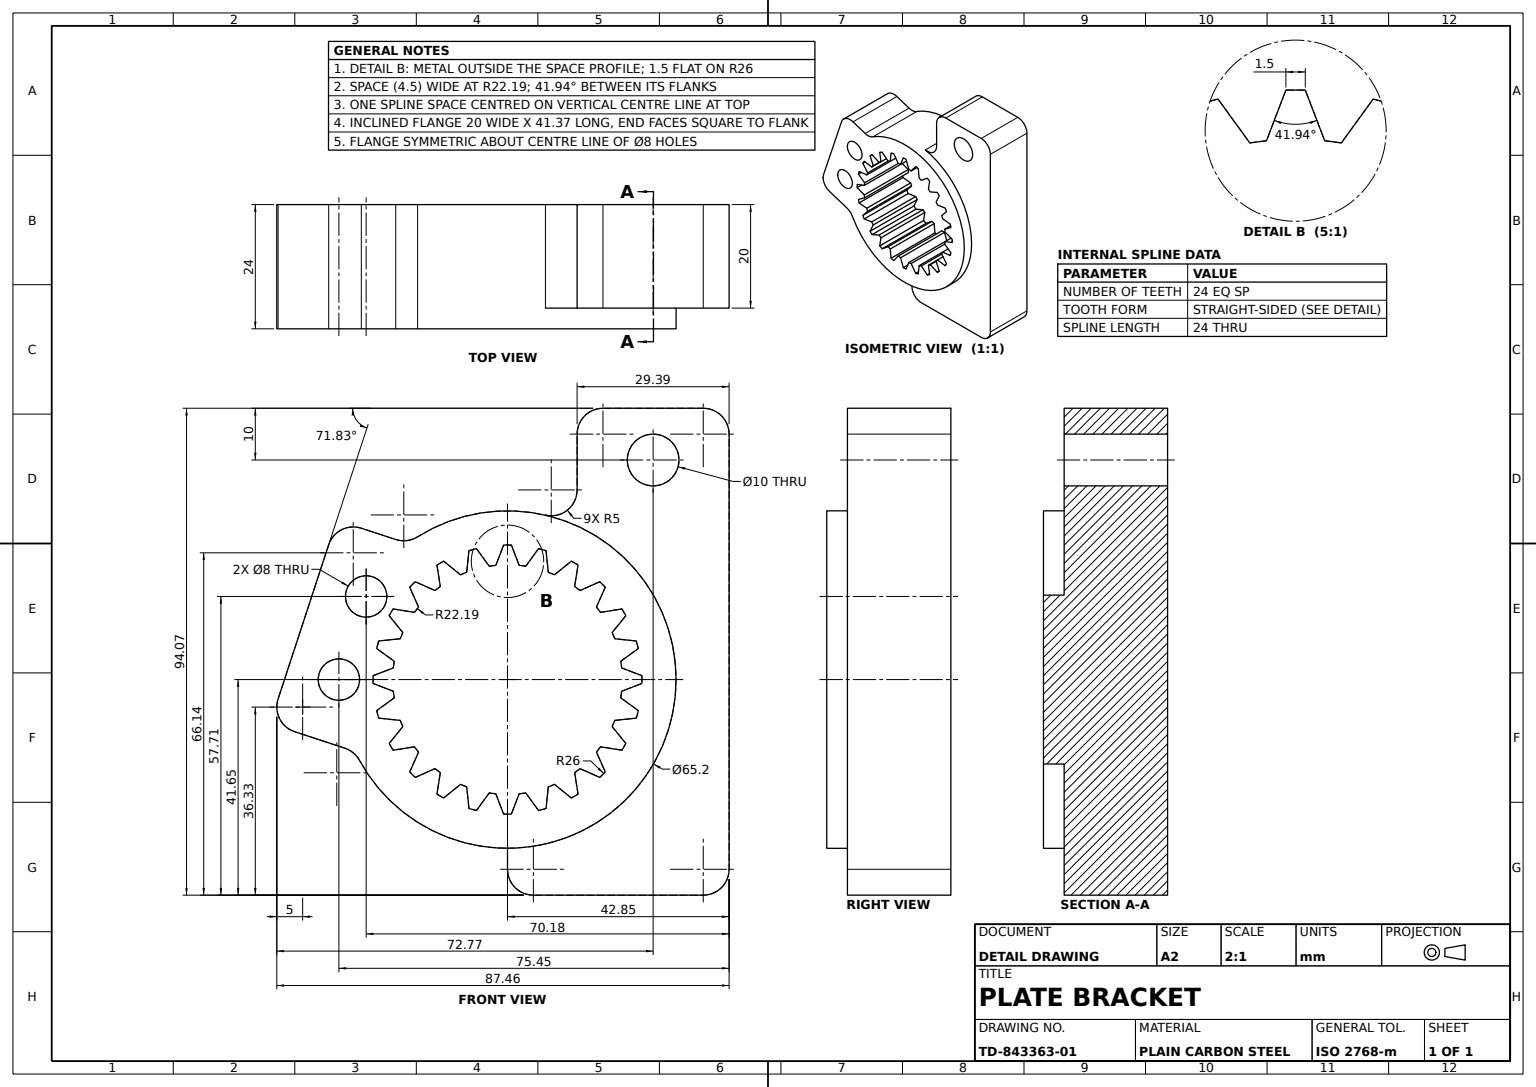
solid
v1 (37.85,52.42,20)
v2 (18.46,52.42,20)
e1 v1 v2 LINE
v3 (13.46,47.42,20)
e2 v2 v3 CIRCLE(AX(P(18.46,47.42,20),D(0,0,1),D(1,0,0)),5)
v4 (13.46,36.63589,20)
e3 v3 v4 LINE
v5 (7.335,31.764096,20)
e4 v4 v5 CIRCLE(AX(P(8.46,36.63589,20),D(0,0,-1),D(1,0,0)),5)
v6 (0,-32.6,20)
e5 v6 v5 CIRCLE(AX(P(0,0,20),D(0,0,1),D(1,0,0)),32.6)
v7 (0,-36.65,20)
e6 v6 v7 LINE
v8 (5,-41.65,20)
e7 v7 v8 CIRCLE(AX(P(5,-36.65,20),D(0,0,1),D(1,0,0)),5)
v9 (37.85,-41.65,20)
e8 v8 v9 LINE
v10 (42.85,-36.65,20)
e9 v9 v10 CIRCLE(AX(P(37.85,-36.65,20),D(0,0,1),D(1,0,0)),5)
v11 (42.85,47.42,20)
e10 v10 v11 LINE
e11 v11 v1 CIRCLE(AX(P(37.85,47.42,20),D(0,0,1),D(1,0,0)),5)
v12 (23.16,42.42,20)
v13 (33.16,42.42,20)
e12 v12 v13 CIRCLE(AX(P(28.16,42.42,20),D(0,0,1),D(1,0,0)),5)
e13 v13 v12 CIRCLE(AX(P(28.16,42.42,20),D(0,0,1),D(1,0,0)),5)
face PLANE(AX(P(0,0,20),D(0,0,1),D(1,0,0))) [e1 e2 e3 e4 -e5 e6 e7 e8 e9 e10 e11] [-e12 -e13]
v14 (-24.909506,7.450939,0)
v15 (-24.909506,7.450939,24)
e14 v14 v15 LINE
v16 (-25.297735,6.00205,24)
e15 v15 v16 CIRCLE(AX(P(0,0,24),D(0,0,1),D(1,0,0)),26)
v17 (-25.297735,6.00205,0)
e16 v17 v16 LINE
e17 v14 v17 CIRCLE(AX(P(0,0,0),D(0,0,1),D(1,0,0)),26)
face CYL(AX(P(0,0,0),D(0,0,1),D(1,0,0)),26) rev [e14 e15 -e16 -e17]
v18 (22.075634,-2.25,0)
v19 (25.98918,-0.75,0)
e18 v18 v19 LINE
v20 (22.075634,-2.25,24)
e19 v18 v20 LINE
v21 (25.98918,-0.75,24)
e20 v20 v21 LINE
e21 v19 v21 LINE
face PLANE(AX(P(3.579582,-9.339241,0),D(0.357895873,-0.933761503,0),D(0.933761503,0.357895873,0))) rev [-e18 e19 e20 -e21]
v22 (-3.540261,-21.905768,0)
v23 (-3.540261,-21.905768,24)
e22 v22 v23 LINE
v24 (-6.00205,-25.297735,0)
e23 v22 v24 LINE
v25 (-6.00205,-25.297735,24)
e24 v24 v25 LINE
e25 v23 v25 LINE
face PLANE(AX(P(8.09455,-5.874784,0),D(-0.809314083,0.587376127,0),D(-0.587376127,-0.809314083,0))) [-e22 e23 e24 -e25]
v26 (-17.99306,12.986374,0)
v27 (-17.99306,12.986374,24)
e26 v26 v27 LINE
v28 (-17.20082,14.01884,0)
e27 v28 v26 CIRCLE(AX(P(0,0,0),D(0,0,1),D(1,0,0)),22.19)
v29 (-17.20082,14.01884,24)
e28 v28 v29 LINE
e29 v29 v27 CIRCLE(AX(P(0,0,24),D(0,0,1),D(1,0,0)),22.19)
face CYL(AX(P(0,0,0),D(0,0,1),D(1,0,0)),22.19) rev [-e26 -e27 e28 e29]
v30 (-0.75,-25.98918,24)
v31 (0.75,-25.98918,24)
e30 v30 v31 CIRCLE(AX(P(0,0,24),D(0,0,1),D(1,0,0)),26)
v32 (0.75,-25.98918,0)
e31 v32 v31 LINE
v33 (-0.75,-25.98918,0)
e32 v33 v32 CIRCLE(AX(P(0,0,0),D(0,0,1),D(1,0,0)),26)
e33 v33 v30 LINE
face CYL(AX(P(0,0,0),D(0,0,1),D(1,0,0)),26) rev [e30 -e31 -e32 e33]
v34 (3.540261,-21.905768,0)
v35 (3.540261,-21.905768,24)
e34 v34 v35 LINE
v36 (2.25,-22.075634,0)
e35 v36 v34 CIRCLE(AX(P(0,0,0),D(0,0,1),D(1,0,0)),22.19)
v37 (2.25,-22.075634,24)
e36 v36 v37 LINE
e37 v37 v35 CIRCLE(AX(P(0,0,24),D(0,0,1),D(1,0,0)),22.19)
face CYL(AX(P(0,0,0),D(0,0,1),D(1,0,0)),22.19) rev [-e34 -e35 e36 e37]
v38 (6.00205,-25.297735,0)
e38 v34 v38 LINE
v39 (6.00205,-25.297735,24)
e39 v35 v39 LINE
e40 v38 v39 LINE
face PLANE(AX(P(-8.09455,-5.874784,0),D(-0.809314083,-0.587376127,0),D(0.587376127,-0.809314083,0))) rev [-e38 e34 e39 -e40]
v40 (0.75,25.98918,0)
v41 (0.75,25.98918,24)
e41 v40 v41 LINE
v42 (2.25,22.075634,0)
e42 v42 v40 LINE
v43 (2.25,22.075634,24)
e43 v42 v43 LINE
e44 v43 v41 LINE
face PLANE(AX(P(9.339241,3.579582,0),D(0.933761503,0.357895873,0),D(-0.357895873,0.933761503,0))) rev [-e41 -e42 e43 e44]
v44 (17.20082,-14.01884,24)
v45 (18.907456,-17.846796,24)
e45 v44 v45 LINE
v46 (17.20082,-14.01884,0)
e46 v46 v44 LINE
v47 (18.907456,-17.846796,0)
e47 v46 v47 LINE
e48 v47 v45 LINE
face PLANE(AX(P(9.134988,4.072694,0),D(-0.913339689,-0.407198492,0),D(0.407198492,-0.913339689,0))) [-e45 -e46 e47 e48]
v48 (13.46,47.42,0)
v49 (18.46,52.42,0)
e49 v48 v49 CIRCLE(AX(P(18.46,47.42,0),D(0,0,-1),D(1,0,0)),5)
e50 v3 v48 LINE
e51 v49 v2 LINE
face CYL(AX(P(18.46,47.42,20),D(0,0,-1),D(-1,0,0)),5) [-e49 -e50 -e2 -e51]
v50 (42.85,-36.65,0)
v51 (37.85,-41.65,0)
e52 v50 v51 CIRCLE(AX(P(37.85,-36.65,0),D(0,0,-1),D(1,0,0)),5)
e53 v10 v50 LINE
e54 v51 v9 LINE
face CYL(AX(P(37.85,-36.65,20),D(0,0,-1),D(-1,0,0)),5) [-e52 -e53 -e9 -e54]
v52 (0,-32.6,0)
e55 v6 v52 LINE
v53 (7.335,31.764096,0)
e56 v5 v53 LINE
v54 (-17.384339,27.577976,0)
e57 v53 v54 CIRCLE(AX(P(0,0,0),D(0,0,1),D(1,0,0)),32.6)
v55 (-17.384339,27.577976,24)
e58 v54 v55 LINE
v56 (-28.619127,-15.611072,24)
e59 v56 v55 CIRCLE(AX(P(0,0,24),D(0,0,1),D(1,0,0)),32.6)
v57 (-28.619127,-15.611072,0)
e60 v56 v57 LINE
e61 v57 v52 CIRCLE(AX(P(0,0,0),D(0,0,1),D(1,0,0)),32.6)
face CYL(AX(P(0,0,24),D(0,0,-1),D(-1,0,0)),32.6) [-e55 e5 e56 e57 e58 -e59 e60 e61]
v58 (7.450939,-24.909506,0)
v59 (7.450939,-24.909506,24)
e62 v58 v59 LINE
e63 v38 v58 CIRCLE(AX(P(0,0,0),D(0,0,1),D(1,0,0)),26)
e64 v39 v59 CIRCLE(AX(P(0,0,24),D(0,0,1),D(1,0,0)),26)
face CYL(AX(P(0,0,0),D(0,0,1),D(1,0,0)),26) rev [-e62 -e63 e40 e64]
v60 (-2.25,22.075634,24)
v61 (-3.540261,21.905768,24)
e65 v60 v61 CIRCLE(AX(P(0,0,24),D(0,0,1),D(1,0,0)),22.19)
v62 (-3.540261,21.905768,0)
e66 v62 v61 LINE
v63 (-2.25,22.075634,0)
e67 v63 v62 CIRCLE(AX(P(0,0,0),D(0,0,1),D(1,0,0)),22.19)
e68 v63 v60 LINE
face CYL(AX(P(0,0,0),D(0,0,1),D(1,0,0)),22.19) rev [e65 -e66 -e67 e68]
v64 (-41.165975,-10.065748,0)
v65 (-44.606804,-5.315066,0)
e69 v64 v65 CIRCLE(AX(P(-39.606804,-5.315066,0),D(0,0,-1),D(1,0,0)),5)
v66 (-41.165975,-10.065748,24)
e70 v66 v64 LINE
v67 (-44.606804,-5.315066,24)
e71 v67 v66 CIRCLE(AX(P(-39.606804,-5.315066,24),D(0,0,1),D(1,0,0)),5)
e72 v67 v65 LINE
face CYL(AX(P(-39.606804,-5.315066,0),D(0,0,-1),D(-1,0,0)),5) [-e69 -e70 -e71 e72]
v68 (-21.609821,27.057044,24)
e73 v55 v68 CIRCLE(AX(P(-20.050649,31.807727,24),D(0,0,-1),D(1,0,0)),5)
v69 (-21.609821,27.057044,0)
e74 v69 v54 CIRCLE(AX(P(-20.050649,31.807727,0),D(0,0,1),D(1,0,0)),5)
e75 v68 v69 LINE
face CYL(AX(P(-20.050649,31.807727,24),D(0,0,-1),D(-1,0,0)),5) rev [-e73 -e58 -e74 -e75]
v70 (-22.075634,2.25,24)
v71 (-25.98918,0.75,24)
e76 v70 v71 LINE
v72 (-25.98918,0.75,0)
e77 v72 v71 LINE
v73 (-22.075634,2.25,0)
e78 v73 v72 LINE
e79 v73 v70 LINE
face PLANE(AX(P(-3.579582,9.339241,0),D(-0.357895873,0.933761503,0),D(-0.933761503,-0.357895873,0))) rev [e76 -e77 -e78 e79]
v74 (-0.75,25.98918,0)
v75 (-0.75,25.98918,24)
e80 v74 v75 LINE
e81 v60 v75 LINE
e82 v63 v74 LINE
face PLANE(AX(P(-9.339241,3.579582,0),D(0.933761503,-0.357895873,0),D(0.357895873,0.933761503,0))) [e80 -e81 -e68 e82]
v76 (22.88229,-12.345071,0)
v77 (22.88229,-12.345071,24)
e83 v76 v77 LINE
v78 (20.24306,-9.08926,24)
e84 v78 v77 LINE
v79 (20.24306,-9.08926,0)
e85 v79 v78 LINE
e86 v79 v76 LINE
face PLANE(AX(P(7.76963,6.298229,0),D(-0.776827669,-0.629713246,0),D(0.629713246,-0.776827669,0))) [e83 -e84 -e85 e86]
v80 (9.08926,20.24306,0)
v81 (9.08926,20.24306,24)
e87 v80 v81 LINE
v82 (12.345071,22.88229,0)
e88 v80 v82 LINE
v83 (12.345071,22.88229,24)
e89 v82 v83 LINE
e90 v81 v83 LINE
face PLANE(AX(P(-6.298229,7.76963,0),D(0.629713246,-0.776827669,0),D(0.776827669,0.629713246,0))) [-e87 e88 e89 -e90]
v84 (25.98918,0.75,0)
v85 (25.98918,0.75,24)
e91 v84 v85 LINE
v86 (26,0,0)
e92 v86 v84 CIRCLE(AX(P(0,0,0),D(0,0,1),D(1,0,0)),26)
v87 (26,0,24)
e93 v86 v87 LINE
e94 v87 v85 CIRCLE(AX(P(0,0,24),D(0,0,1),D(1,0,0)),26)
face CYL(AX(P(0,0,0),D(0,0,1),D(1,0,0)),26) rev [-e91 -e92 e93 e94]
v88 (-20.741082,7.886928,0)
v89 (-20.741082,7.886928,24)
e95 v88 v89 LINE
e96 v89 v15 LINE
e97 v88 v14 LINE
face PLANE(AX(P(-1.040437,9.947478,0),D(-0.104025606,0.994574619,0),D(-0.994574619,-0.104025606,0))) rev [e95 e96 -e14 -e97]
v90 (7.886928,20.741082,0)
v91 (7.886928,20.741082,24)
e98 v90 v91 LINE
e99 v80 v90 CIRCLE(AX(P(0,0,0),D(0,0,1),D(1,0,0)),22.19)
e100 v81 v91 CIRCLE(AX(P(0,0,24),D(0,0,1),D(1,0,0)),22.19)
face CYL(AX(P(0,0,0),D(0,0,1),D(1,0,0)),22.19) rev [-e98 -e99 e87 e100]
v92 (20.741082,-7.886928,0)
v93 (24.909506,-7.450939,0)
e101 v92 v93 LINE
v94 (20.741082,-7.886928,24)
e102 v92 v94 LINE
v95 (24.909506,-7.450939,24)
e103 v94 v95 LINE
e104 v93 v95 LINE
face PLANE(AX(P(1.040437,-9.947478,0),D(0.104025606,-0.994574619,0),D(0.994574619,0.104025606,0))) rev [-e101 e102 e103 -e104]
v96 (12.345071,-22.88229,0)
v97 (12.345071,-22.88229,24)
e105 v96 v97 LINE
v98 (13.644109,-22.13229,24)
e106 v97 v98 CIRCLE(AX(P(0,0,24),D(0,0,1),D(1,0,0)),26)
v99 (13.644109,-22.13229,0)
e107 v99 v98 LINE
e108 v96 v99 CIRCLE(AX(P(0,0,0),D(0,0,1),D(1,0,0)),26)
face CYL(AX(P(0,0,0),D(0,0,1),D(1,0,0)),26) rev [e105 e106 -e107 -e108]
v100 (22.13229,-13.644109,0)
e109 v100 v76 CIRCLE(AX(P(0,0,0),D(0,0,1),D(1,0,0)),26)
v101 (22.13229,-13.644109,24)
e110 v100 v101 LINE
e111 v101 v77 CIRCLE(AX(P(0,0,24),D(0,0,1),D(1,0,0)),26)
face CYL(AX(P(0,0,0),D(0,0,1),D(1,0,0)),26) rev [-e83 -e109 e110 e111]
v102 (9.08926,-20.24306,0)
e112 v102 v96 LINE
v103 (9.08926,-20.24306,24)
e113 v102 v103 LINE
e114 v103 v97 LINE
face PLANE(AX(P(-6.298229,-7.76963,0),D(-0.629713246,-0.776827669,0),D(0.776827669,-0.629713246,0))) rev [-e105 -e112 e113 e114]
v104 (-14.01884,17.20082,0)
v105 (-14.01884,17.20082,24)
e115 v104 v105 LINE
v106 (-12.986374,17.99306,0)
e116 v106 v104 CIRCLE(AX(P(0,0,0),D(0,0,1),D(1,0,0)),22.19)
v107 (-12.986374,17.99306,24)
e117 v106 v107 LINE
e118 v107 v105 CIRCLE(AX(P(0,0,24),D(0,0,1),D(1,0,0)),22.19)
face CYL(AX(P(0,0,0),D(0,0,1),D(1,0,0)),22.19) rev [-e115 -e116 e117 e118]
v108 (12.986374,17.99306,0)
v109 (12.986374,17.99306,24)
e119 v108 v109 LINE
v110 (13.644109,22.13229,24)
e120 v109 v110 LINE
v111 (13.644109,22.13229,0)
e121 v111 v110 LINE
e122 v108 v111 LINE
face PLANE(AX(P(9.877811,-1.569612,0),D(0.987609119,-0.156933833,0),D(0.156933833,0.987609119,0))) rev [e119 e120 -e121 -e122]
e123 v41 v75 CIRCLE(AX(P(0,0,24),D(0,0,1),D(1,0,0)),26)
e124 v40 v74 CIRCLE(AX(P(0,0,0),D(0,0,1),D(1,0,0)),26)
face CYL(AX(P(0,0,0),D(0,0,1),D(1,0,0)),26) rev [e123 -e80 -e124 e41]
v112 (21.905768,-3.540261,24)
e125 v112 v20 CIRCLE(AX(P(0,0,24),D(0,0,1),D(1,0,0)),22.19)
v113 (21.905768,-3.540261,0)
e126 v113 v18 CIRCLE(AX(P(0,0,0),D(0,0,1),D(1,0,0)),22.19)
e127 v113 v112 LINE
face CYL(AX(P(0,0,0),D(0,0,1),D(1,0,0)),22.19) rev [e125 -e19 -e126 e127]
v114 (-23.33,16.057307,24)
v115 (-31.33,16.057307,24)
e128 v114 v115 CIRCLE(AX(P(-27.33,16.057307,24),D(0,0,1),D(1,0,0)),4)
v116 (-31.33,16.057307,0)
e129 v116 v115 LINE
v117 (-23.33,16.057307,0)
e130 v117 v116 CIRCLE(AX(P(-27.33,16.057307,0),D(0,0,1),D(1,0,0)),4)
e131 v117 v114 LINE
face CYL(AX(P(-27.33,16.057307,0),D(0,0,1),D(1,0,0)),4) rev [e128 -e129 -e130 e131]
v118 (-22.88229,-12.345071,0)
v119 (-22.13229,-13.644109,0)
e132 v118 v119 CIRCLE(AX(P(0,0,0),D(0,0,1),D(1,0,0)),26)
v120 (-22.88229,-12.345071,24)
e133 v118 v120 LINE
v121 (-22.13229,-13.644109,24)
e134 v120 v121 CIRCLE(AX(P(0,0,24),D(0,0,1),D(1,0,0)),26)
e135 v119 v121 LINE
face CYL(AX(P(0,0,0),D(0,0,1),D(1,0,0)),26) rev [-e132 e133 e134 -e135]
v122 (22.075634,2.25,24)
e136 v122 v85 LINE
v123 (22.075634,2.25,0)
e137 v123 v122 LINE
e138 v123 v84 LINE
face PLANE(AX(P(3.579582,9.339241,0),D(-0.357895873,-0.933761503,0),D(0.933761503,-0.357895873,0))) [e91 -e136 -e137 e138]
v124 (20.24306,9.08926,0)
v125 (22.88229,12.345071,0)
e139 v124 v125 LINE
v126 (20.24306,9.08926,24)
e140 v124 v126 LINE
v127 (22.88229,12.345071,24)
e141 v126 v127 LINE
e142 v125 v127 LINE
face PLANE(AX(P(7.76963,-6.298229,0),D(0.776827669,-0.629713246,0),D(0.629713246,0.776827669,0))) rev [-e139 e140 e141 -e142]
v128 (12.986374,-17.99306,0)
v129 (14.01884,-17.20082,0)
e143 v128 v129 CIRCLE(AX(P(0,0,0),D(0,0,1),D(1,0,0)),22.19)
v130 (12.986374,-17.99306,24)
e144 v128 v130 LINE
v131 (14.01884,-17.20082,24)
e145 v130 v131 CIRCLE(AX(P(0,0,24),D(0,0,1),D(1,0,0)),22.19)
e146 v129 v131 LINE
face CYL(AX(P(0,0,0),D(0,0,1),D(1,0,0)),22.19) rev [-e143 e144 e145 -e146]
v132 (25.297735,-6.00205,24)
e147 v112 v132 LINE
v133 (25.297735,-6.00205,0)
e148 v113 v133 LINE
e149 v133 v132 LINE
face PLANE(AX(P(5.874784,8.09455,0),D(-0.587376127,-0.809314083,0),D(0.809314083,-0.587376127,0))) [-e147 -e127 e148 e149]
v134 (-17.99306,-12.986374,0)
v135 (-17.99306,-12.986374,24)
e150 v134 v135 LINE
v136 (-17.20082,-14.01884,24)
e151 v135 v136 CIRCLE(AX(P(0,0,24),D(0,0,1),D(1,0,0)),22.19)
v137 (-17.20082,-14.01884,0)
e152 v137 v136 LINE
e153 v134 v137 CIRCLE(AX(P(0,0,0),D(0,0,1),D(1,0,0)),22.19)
face CYL(AX(P(0,0,0),D(0,0,1),D(1,0,0)),22.19) rev [e150 e151 -e152 -e153]
v138 (-13.644109,-22.13229,24)
v139 (-12.345071,-22.88229,24)
e154 v138 v139 CIRCLE(AX(P(0,0,24),D(0,0,1),D(1,0,0)),26)
v140 (-12.345071,-22.88229,0)
e155 v140 v139 LINE
v141 (-13.644109,-22.13229,0)
e156 v141 v140 CIRCLE(AX(P(0,0,0),D(0,0,1),D(1,0,0)),26)
e157 v141 v138 LINE
face CYL(AX(P(0,0,0),D(0,0,1),D(1,0,0)),26) rev [e154 -e155 -e156 e157]
v142 (7.450939,24.909506,24)
e158 v91 v142 LINE
v143 (7.450939,24.909506,0)
e159 v143 v142 LINE
e160 v90 v143 LINE
face PLANE(AX(P(9.947478,1.040437,0),D(0.994574619,0.104025606,0),D(-0.104025606,0.994574619,0))) rev [e158 -e159 -e160 e98]
e161 v111 v82 CIRCLE(AX(P(0,0,0),D(0,0,1),D(1,0,0)),26)
e162 v110 v83 CIRCLE(AX(P(0,0,24),D(0,0,1),D(1,0,0)),26)
face CYL(AX(P(0,0,0),D(0,0,1),D(1,0,0)),26) rev [-e89 -e161 e121 e162]
v144 (-21.905768,-3.540261,0)
v145 (-21.905768,-3.540261,24)
e163 v144 v145 LINE
v146 (-22.075634,-2.25,0)
e164 v146 v144 CIRCLE(AX(P(0,0,0),D(0,0,1),D(1,0,0)),22.19)
v147 (-22.075634,-2.25,24)
e165 v146 v147 LINE
e166 v147 v145 CIRCLE(AX(P(0,0,24),D(0,0,1),D(1,0,0)),22.19)
face CYL(AX(P(0,0,0),D(0,0,1),D(1,0,0)),22.19) rev [-e163 -e164 e165 e166]
v148 (-7.886928,-20.741082,24)
v149 (-7.450939,-24.909506,24)
e167 v148 v149 LINE
v150 (-7.450939,-24.909506,0)
e168 v150 v149 LINE
v151 (-7.886928,-20.741082,0)
e169 v151 v150 LINE
e170 v151 v148 LINE
face PLANE(AX(P(-9.947478,-1.040437,0),D(-0.994574619,-0.104025606,0),D(0.104025606,-0.994574619,0))) rev [e167 -e168 -e169 e170]
v152 (-17.846796,18.907456,0)
v153 (-18.907456,17.846796,0)
e171 v152 v153 CIRCLE(AX(P(0,0,0),D(0,0,1),D(1,0,0)),26)
v154 (-17.846796,18.907456,24)
e172 v152 v154 LINE
v155 (-18.907456,17.846796,24)
e173 v154 v155 CIRCLE(AX(P(0,0,24),D(0,0,1),D(1,0,0)),26)
e174 v153 v155 LINE
face CYL(AX(P(0,0,0),D(0,0,1),D(1,0,0)),26) rev [-e171 e172 e173 -e174]
v156 (-22.13229,13.644109,24)
v157 (-22.88229,12.345071,24)
e175 v156 v157 CIRCLE(AX(P(0,0,24),D(0,0,1),D(1,0,0)),26)
v158 (-22.88229,12.345071,0)
e176 v158 v157 LINE
v159 (-22.13229,13.644109,0)
e177 v159 v158 CIRCLE(AX(P(0,0,0),D(0,0,1),D(1,0,0)),26)
e178 v159 v156 LINE
face CYL(AX(P(0,0,0),D(0,0,1),D(1,0,0)),26) rev [e175 -e176 -e177 e178]
e179 v95 v132 CIRCLE(AX(P(0,0,24),D(0,0,1),D(1,0,0)),26)
e180 v93 v133 CIRCLE(AX(P(0,0,0),D(0,0,1),D(1,0,0)),26)
face CYL(AX(P(0,0,0),D(0,0,1),D(1,0,0)),26) rev [e104 e179 -e149 -e180]
v160 (17.99306,-12.986374,0)
e181 v160 v100 LINE
v161 (17.99306,-12.986374,24)
e182 v160 v161 LINE
e183 v161 v101 LINE
face PLANE(AX(P(-1.569612,-9.877811,0),D(-0.156933833,-0.987609119,0),D(0.987609119,-0.156933833,0))) rev [-e181 e182 e183 -e110]
v162 (-14.01884,-17.20082,24)
v163 (-17.846796,-18.907456,24)
e184 v162 v163 LINE
v164 (-14.01884,-17.20082,0)
e185 v164 v162 LINE
v165 (-17.846796,-18.907456,0)
e186 v164 v165 LINE
e187 v165 v163 LINE
face PLANE(AX(P(4.072694,-9.134988,0),D(-0.407198492,0.913339689,0),D(-0.913339689,-0.407198492,0))) [-e184 -e185 e186 e187]
v166 (-28.26539,29.241398,0)
v167 (-28.26539,29.241398,24)
e188 v166 v167 LINE
e189 v167 v68 LINE
e190 v166 v69 LINE
face PLANE(AX(P(5.915248,18.02333,0),D(-0.31183432,-0.950136494,0),D(0.950136494,-0.31183432,0))) rev [e188 e189 e75 -e190]
v168 (13.46,36.63589,0)
e191 v53 v168 CIRCLE(AX(P(8.46,36.63589,0),D(0,0,1),D(1,0,0)),5)
e192 v48 v168 LINE
v169 (37.85,52.42,0)
e193 v169 v49 LINE
v170 (42.85,47.42,0)
e194 v169 v170 CIRCLE(AX(P(37.85,47.42,0),D(0,0,-1),D(1,0,0)),5)
e195 v50 v170 LINE
v171 (5,-41.65,0)
e196 v171 v51 LINE
v172 (0,-36.65,0)
e197 v171 v172 CIRCLE(AX(P(5,-36.65,0),D(0,0,-1),D(1,0,0)),5)
e198 v52 v172 LINE
v173 (-31.449392,-13.254726,0)
e199 v57 v173 CIRCLE(AX(P(-33.008563,-18.005409,0),D(0,0,1),D(1,0,0)),5)
e200 v64 v173 LINE
v174 (-44.357486,-3.755894,0)
e201 v65 v174 CIRCLE(AX(P(-39.606804,-5.315066,0),D(0,0,-1),D(1,0,0)),5)
v175 (-34.575244,26.049887,0)
e202 v174 v175 LINE
e203 v175 v166 CIRCLE(AX(P(-29.824561,24.490716,0),D(0,0,-1),D(1,0,0)),5)
e204 v116 v117 CIRCLE(AX(P(-27.33,16.057307,0),D(0,0,1),D(1,0,0)),4)
v176 (-36.6,0,0)
v177 (-28.6,0,0)
e205 v176 v177 CIRCLE(AX(P(-32.6,0,0),D(0,0,1),D(1,0,0)),4)
e206 v177 v176 CIRCLE(AX(P(-32.6,0,0),D(0,0,1),D(1,0,0)),4)
v178 (-25.98918,-0.75,0)
e207 v72 v178 CIRCLE(AX(P(0,0,0),D(0,0,1),D(1,0,0)),26)
e208 v146 v178 LINE
v179 (-25.297735,-6.00205,0)
e209 v144 v179 LINE
v180 (-24.909506,-7.450939,0)
e210 v179 v180 CIRCLE(AX(P(0,0,0),D(0,0,1),D(1,0,0)),26)
v181 (-20.741082,-7.886928,0)
e211 v181 v180 LINE
v182 (-20.24306,-9.08926,0)
e212 v181 v182 CIRCLE(AX(P(0,0,0),D(0,0,1),D(1,0,0)),22.19)
e213 v182 v118 LINE
e214 v134 v119 LINE
v183 (-18.907456,-17.846796,0)
e215 v137 v183 LINE
e216 v183 v165 CIRCLE(AX(P(0,0,0),D(0,0,1),D(1,0,0)),26)
v184 (-12.986374,-17.99306,0)
e217 v164 v184 CIRCLE(AX(P(0,0,0),D(0,0,1),D(1,0,0)),22.19)
e218 v184 v141 LINE
v185 (-9.08926,-20.24306,0)
e219 v185 v140 LINE
e220 v185 v151 CIRCLE(AX(P(0,0,0),D(0,0,1),D(1,0,0)),22.19)
e221 v150 v24 CIRCLE(AX(P(0,0,0),D(0,0,1),D(1,0,0)),26)
v186 (-2.25,-22.075634,0)
e222 v22 v186 CIRCLE(AX(P(0,0,0),D(0,0,1),D(1,0,0)),22.19)
e223 v186 v33 LINE
e224 v36 v32 LINE
v187 (7.886928,-20.741082,0)
e225 v187 v58 LINE
e226 v187 v102 CIRCLE(AX(P(0,0,0),D(0,0,1),D(1,0,0)),22.19)
e227 v128 v99 LINE
v188 (17.846796,-18.907456,0)
e228 v129 v188 LINE
e229 v188 v47 CIRCLE(AX(P(0,0,0),D(0,0,1),D(1,0,0)),26)
e230 v46 v160 CIRCLE(AX(P(0,0,0),D(0,0,1),D(1,0,0)),22.19)
e231 v79 v92 CIRCLE(AX(P(0,0,0),D(0,0,1),D(1,0,0)),22.19)
e232 v19 v86 CIRCLE(AX(P(0,0,0),D(0,0,1),D(1,0,0)),26)
v189 (21.905768,3.540261,0)
e233 v123 v189 CIRCLE(AX(P(0,0,0),D(0,0,1),D(1,0,0)),22.19)
v190 (25.297735,6.00205,0)
e234 v189 v190 LINE
v191 (24.909506,7.450939,0)
e235 v190 v191 CIRCLE(AX(P(0,0,0),D(0,0,1),D(1,0,0)),26)
v192 (20.741082,7.886928,0)
e236 v192 v191 LINE
e237 v192 v124 CIRCLE(AX(P(0,0,0),D(0,0,1),D(1,0,0)),22.19)
v193 (22.13229,13.644109,0)
e238 v125 v193 CIRCLE(AX(P(0,0,0),D(0,0,1),D(1,0,0)),26)
v194 (17.99306,12.986374,0)
e239 v194 v193 LINE
v195 (17.20082,14.01884,0)
e240 v194 v195 CIRCLE(AX(P(0,0,0),D(0,0,1),D(1,0,0)),22.19)
v196 (18.907456,17.846796,0)
e241 v195 v196 LINE
v197 (17.846796,18.907456,0)
e242 v196 v197 CIRCLE(AX(P(0,0,0),D(0,0,1),D(1,0,0)),26)
v198 (14.01884,17.20082,0)
e243 v198 v197 LINE
e244 v198 v108 CIRCLE(AX(P(0,0,0),D(0,0,1),D(1,0,0)),22.19)
v199 (6.00205,25.297735,0)
e245 v143 v199 CIRCLE(AX(P(0,0,0),D(0,0,1),D(1,0,0)),26)
v200 (3.540261,21.905768,0)
e246 v200 v199 LINE
e247 v200 v42 CIRCLE(AX(P(0,0,0),D(0,0,1),D(1,0,0)),22.19)
v201 (-6.00205,25.297735,0)
e248 v62 v201 LINE
v202 (-7.450939,24.909506,0)
e249 v201 v202 CIRCLE(AX(P(0,0,0),D(0,0,1),D(1,0,0)),26)
v203 (-7.886928,20.741082,0)
e250 v203 v202 LINE
v204 (-9.08926,20.24306,0)
e251 v203 v204 CIRCLE(AX(P(0,0,0),D(0,0,1),D(1,0,0)),22.19)
v205 (-12.345071,22.88229,0)
e252 v204 v205 LINE
v206 (-13.644109,22.13229,0)
e253 v205 v206 CIRCLE(AX(P(0,0,0),D(0,0,1),D(1,0,0)),26)
e254 v106 v206 LINE
e255 v104 v152 LINE
e256 v28 v153 LINE
e257 v26 v159 LINE
v207 (-20.24306,9.08926,0)
e258 v207 v158 LINE
e259 v207 v88 CIRCLE(AX(P(0,0,0),D(0,0,1),D(1,0,0)),22.19)
v208 (-21.905768,3.540261,0)
e260 v208 v17 LINE
e261 v208 v73 CIRCLE(AX(P(0,0,0),D(0,0,1),D(1,0,0)),22.19)
v209 (33.16,42.42,0)
v210 (23.16,42.42,0)
e262 v209 v210 CIRCLE(AX(P(28.16,42.42,0),D(0,0,1),D(1,0,0)),5)
e263 v210 v209 CIRCLE(AX(P(28.16,42.42,0),D(0,0,1),D(1,0,0)),5)
face PLANE(AX(P(0,0,0),D(0,0,1),D(1,0,0))) rev [-e57 e191 -e192 e49 -e193 e194 -e195 e52 -e196 e197 -e198 -e61 e199 -e200 e69 e201 e202 e203 e190 e74] [e204 e130] [e205 e206] [e207 -e208 e164 e209 e210 -e211 e212 e213 e132 -e214 e153 e215 e216 -e186 e217 e218 e156 -e219 e220 e169 e221 -e23 e222 e223 e32 -e224 e35 e38 e63 -e225 e226 e112 e108 -e227 e143 e228 e229 -e47 e230 e181 e109 -e86 e231 e101 e180 -e148 e126 e18 e232 e92 -e138 e233 e234 e235 -e236 e237 e139 e238 -e239 e240 e241 e242 -e243 e244 e122 e161 -e88 e99 e160 e245 -e246 e247 e42 e124 -e82 e67 e248 e249 -e250 e251 e252 e253 -e254 e116 e255 e171 -e256 e27 e257 e177 -e258 e259 e97 e17 -e260 e261 e78] [e262 e263]
v211 (-20.24306,9.08926,24)
e264 v207 v211 LINE
e265 v211 v89 CIRCLE(AX(P(0,0,24),D(0,0,1),D(1,0,0)),22.19)
face CYL(AX(P(0,0,0),D(0,0,1),D(1,0,0)),22.19) rev [-e95 -e259 e264 e265]
e266 v115 v114 CIRCLE(AX(P(-27.33,16.057307,24),D(0,0,1),D(1,0,0)),4)
face CYL(AX(P(-27.33,16.057307,0),D(0,0,1),D(1,0,0)),4) rev [-e131 -e204 e129 e266]
v212 (17.20082,14.01884,24)
e267 v195 v212 LINE
v213 (18.907456,17.846796,24)
e268 v212 v213 LINE
e269 v196 v213 LINE
face PLANE(AX(P(9.134988,-4.072694,0),D(0.913339689,-0.407198492,0),D(0.407198492,0.913339689,0))) rev [-e241 e267 e268 -e269]
e270 v211 v157 LINE
face PLANE(AX(P(-7.76963,-6.298229,0),D(0.776827669,0.629713246,0),D(-0.629713246,0.776827669,0))) [-e270 -e264 e258 e176]
e271 v172 v7 LINE
e272 v8 v171 LINE
face CYL(AX(P(5,-36.65,20),D(0,0,-1),D(-1,0,0)),5) [-e7 -e271 -e197 -e272]
v214 (17.99306,12.986374,24)
e273 v194 v214 LINE
e274 v214 v212 CIRCLE(AX(P(0,0,24),D(0,0,1),D(1,0,0)),22.19)
face CYL(AX(P(0,0,0),D(0,0,1),D(1,0,0)),22.19) rev [-e267 -e240 e273 e274]
v215 (-28.6,0,24)
v216 (-36.6,0,24)
e275 v215 v216 CIRCLE(AX(P(-32.6,0,24),D(0,0,1),D(1,0,0)),4)
e276 v216 v215 CIRCLE(AX(P(-32.6,0,24),D(0,0,1),D(1,0,0)),4)
e277 v44 v161 CIRCLE(AX(P(0,0,24),D(0,0,1),D(1,0,0)),22.19)
v217 (17.846796,-18.907456,24)
e278 v217 v45 CIRCLE(AX(P(0,0,24),D(0,0,1),D(1,0,0)),26)
e279 v131 v217 LINE
e280 v130 v98 LINE
v218 (7.886928,-20.741082,24)
e281 v218 v103 CIRCLE(AX(P(0,0,24),D(0,0,1),D(1,0,0)),22.19)
e282 v218 v59 LINE
e283 v37 v31 LINE
v219 (-2.25,-22.075634,24)
e284 v219 v30 LINE
e285 v23 v219 CIRCLE(AX(P(0,0,24),D(0,0,1),D(1,0,0)),22.19)
e286 v149 v25 CIRCLE(AX(P(0,0,24),D(0,0,1),D(1,0,0)),26)
v220 (-9.08926,-20.24306,24)
e287 v220 v148 CIRCLE(AX(P(0,0,24),D(0,0,1),D(1,0,0)),22.19)
e288 v220 v139 LINE
v221 (-12.986374,-17.99306,24)
e289 v221 v138 LINE
e290 v162 v221 CIRCLE(AX(P(0,0,24),D(0,0,1),D(1,0,0)),22.19)
v222 (-18.907456,-17.846796,24)
e291 v222 v163 CIRCLE(AX(P(0,0,24),D(0,0,1),D(1,0,0)),26)
e292 v136 v222 LINE
e293 v135 v121 LINE
v223 (-20.24306,-9.08926,24)
e294 v223 v120 LINE
v224 (-20.741082,-7.886928,24)
e295 v224 v223 CIRCLE(AX(P(0,0,24),D(0,0,1),D(1,0,0)),22.19)
v225 (-24.909506,-7.450939,24)
e296 v224 v225 LINE
v226 (-25.297735,-6.00205,24)
e297 v226 v225 CIRCLE(AX(P(0,0,24),D(0,0,1),D(1,0,0)),26)
e298 v145 v226 LINE
v227 (-25.98918,-0.75,24)
e299 v147 v227 LINE
e300 v71 v227 CIRCLE(AX(P(0,0,24),D(0,0,1),D(1,0,0)),26)
v228 (-21.905768,3.540261,24)
e301 v228 v70 CIRCLE(AX(P(0,0,24),D(0,0,1),D(1,0,0)),22.19)
e302 v228 v16 LINE
e303 v27 v156 LINE
e304 v29 v155 LINE
e305 v105 v154 LINE
v229 (-13.644109,22.13229,24)
e306 v107 v229 LINE
v230 (-12.345071,22.88229,24)
e307 v230 v229 CIRCLE(AX(P(0,0,24),D(0,0,1),D(1,0,0)),26)
v231 (-9.08926,20.24306,24)
e308 v231 v230 LINE
v232 (-7.886928,20.741082,24)
e309 v232 v231 CIRCLE(AX(P(0,0,24),D(0,0,1),D(1,0,0)),22.19)
v233 (-7.450939,24.909506,24)
e310 v232 v233 LINE
v234 (-6.00205,25.297735,24)
e311 v234 v233 CIRCLE(AX(P(0,0,24),D(0,0,1),D(1,0,0)),26)
e312 v61 v234 LINE
v235 (3.540261,21.905768,24)
e313 v235 v43 CIRCLE(AX(P(0,0,24),D(0,0,1),D(1,0,0)),22.19)
v236 (6.00205,25.297735,24)
e314 v235 v236 LINE
e315 v142 v236 CIRCLE(AX(P(0,0,24),D(0,0,1),D(1,0,0)),26)
v237 (14.01884,17.20082,24)
e316 v237 v109 CIRCLE(AX(P(0,0,24),D(0,0,1),D(1,0,0)),22.19)
v238 (17.846796,18.907456,24)
e317 v237 v238 LINE
e318 v213 v238 CIRCLE(AX(P(0,0,24),D(0,0,1),D(1,0,0)),26)
v239 (22.13229,13.644109,24)
e319 v214 v239 LINE
e320 v127 v239 CIRCLE(AX(P(0,0,24),D(0,0,1),D(1,0,0)),26)
v240 (20.741082,7.886928,24)
e321 v240 v126 CIRCLE(AX(P(0,0,24),D(0,0,1),D(1,0,0)),22.19)
v241 (24.909506,7.450939,24)
e322 v240 v241 LINE
v242 (25.297735,6.00205,24)
e323 v242 v241 CIRCLE(AX(P(0,0,24),D(0,0,1),D(1,0,0)),26)
v243 (21.905768,3.540261,24)
e324 v243 v242 LINE
e325 v122 v243 CIRCLE(AX(P(0,0,24),D(0,0,1),D(1,0,0)),22.19)
e326 v21 v87 CIRCLE(AX(P(0,0,24),D(0,0,1),D(1,0,0)),26)
e327 v78 v94 CIRCLE(AX(P(0,0,24),D(0,0,1),D(1,0,0)),22.19)
v244 (-44.357486,-3.755894,24)
v245 (-34.575244,26.049887,24)
e328 v244 v245 LINE
e329 v244 v67 CIRCLE(AX(P(-39.606804,-5.315066,24),D(0,0,1),D(1,0,0)),5)
v246 (-31.449392,-13.254726,24)
e330 v66 v246 LINE
e331 v246 v56 CIRCLE(AX(P(-33.008563,-18.005409,24),D(0,0,-1),D(1,0,0)),5)
e332 v167 v245 CIRCLE(AX(P(-29.824561,24.490716,24),D(0,0,1),D(1,0,0)),5)
face PLANE(AX(P(0,0,24),D(0,0,1),D(1,0,0))) [-e128 -e266] [-e275 -e276] [-e277 e45 -e278 -e279 -e145 e280 -e106 -e114 -e281 e282 -e64 -e39 -e37 e283 -e30 -e284 -e285 e25 -e286 -e167 -e287 e288 -e154 -e289 -e290 e184 -e291 -e292 -e151 e293 -e134 -e294 -e295 e296 -e297 -e298 -e166 e299 -e300 -e76 -e301 e302 -e15 -e96 -e265 e270 -e175 -e303 -e29 e304 -e173 -e305 -e118 e306 -e307 -e308 -e309 e310 -e311 -e312 -e65 e81 -e123 -e44 -e313 e314 -e315 -e158 -e100 e90 -e162 -e120 -e316 e317 -e318 -e268 -e274 e319 -e320 -e141 -e321 e322 -e323 -e324 -e325 e136 -e94 -e326 -e20 -e125 e147 -e179 -e103 -e327 e84 -e111 -e183] [-e328 e329 e71 e330 e331 e59 e73 -e189 e332]
e333 v181 v224 LINE
e334 v180 v225 LINE
face PLANE(AX(P(-1.040437,-9.947478,0),D(0.104025606,0.994574619,0),D(-0.994574619,0.104025606,0))) [-e333 e211 e334 -e296]
face PLANE(AX(P(0,-41.65,20),D(0,1,0),D(0,0,1))) rev [-e8 e272 e196 e54]
e335 v200 v235 LINE
face CYL(AX(P(0,0,0),D(0,0,1),D(1,0,0)),22.19) rev [-e247 e335 e313 -e43]
face PLANE(AX(P(9.339241,-3.579582,0),D(-0.933761503,0.357895873,0),D(-0.357895873,-0.933761503,0))) [e224 e31 -e283 -e36]
e336 v184 v221 LINE
face CYL(AX(P(0,0,0),D(0,0,1),D(1,0,0)),22.19) rev [e185 e290 -e336 -e217]
e337 v202 v233 LINE
e338 v201 v234 LINE
face CYL(AX(P(0,0,0),D(0,0,1),D(1,0,0)),26) rev [-e337 -e249 e338 e311]
e339 v193 v239 LINE
face CYL(AX(P(0,0,0),D(0,0,1),D(1,0,0)),26) rev [e142 e320 -e339 -e238]
face PLANE(AX(P(-9.134988,-4.072694,0),D(0.913339689,0.407198492,0),D(-0.407198492,0.913339689,0))) [-e28 e256 e174 -e304]
e340 v183 v222 LINE
face PLANE(AX(P(-9.134988,4.072694,0),D(-0.913339689,0.407198492,0),D(-0.407198492,-0.913339689,0))) rev [-e215 e152 e292 -e340]
face PLANE(AX(P(8.09455,5.874784,0),D(0.809314083,0.587376127,0),D(-0.587376127,0.809314083,0))) rev [-e338 -e248 e66 e312]
face CYL(AX(P(0,0,0),D(0,0,1),D(1,0,0)),22.19) rev [-e230 e46 e277 -e182]
e341 v185 v220 LINE
face PLANE(AX(P(6.298229,-7.76963,0),D(-0.629713246,0.776827669,0),D(-0.776827669,-0.629713246,0))) [-e341 e219 e155 -e288]
face CYL(AX(P(0,0,0),D(0,0,1),D(1,0,0)),26) rev [e291 -e187 -e216 e340]
e342 v174 v244 LINE
face CYL(AX(P(-39.606804,-5.315066,0),D(0,0,-1),D(-1,0,0)),5) [-e72 -e329 -e342 -e201]
e343 v188 v217 LINE
face CYL(AX(P(0,0,0),D(0,0,1),D(1,0,0)),26) rev [e278 -e48 -e229 e343]
e344 v199 v236 LINE
face PLANE(AX(P(-8.09455,5.874784,0),D(0.809314083,-0.587376127,0),D(0.587376127,0.809314083,0))) [-e335 e246 e344 -e314]
face PLANE(AX(P(1.569612,-9.877811,0),D(-0.156933833,0.987609119,0),D(-0.987609119,-0.156933833,0))) [-e150 e214 e135 -e293]
e345 v206 v229 LINE
e346 v205 v230 LINE
face CYL(AX(P(0,0,0),D(0,0,1),D(1,0,0)),26) rev [-e345 -e253 e346 e307]
e347 v170 v11 LINE
face PLANE(AX(P(42.85,0,20),D(-1,0,0),D(0,0,1))) rev [e53 e195 e347 -e10]
face CYL(AX(P(0,0,0),D(0,0,1),D(1,0,0)),26) rev [e21 e326 -e93 -e232]
e348 v182 v223 LINE
face PLANE(AX(P(-7.76963,6.298229,0),D(-0.776827669,0.629713246,0),D(-0.629713246,-0.776827669,0))) rev [e348 e294 -e133 -e213]
face CYL(AX(P(0,0,0),D(0,0,1),D(1,0,0)),22.19) rev [e85 e327 -e102 -e231]
e349 v168 v4 LINE
face CYL(AX(P(8.46,36.63589,24),D(0,0,-1),D(-1,0,0)),5) rev [-e4 -e349 -e191 -e56]
e350 v179 v226 LINE
face PLANE(AX(P(-5.874784,8.09455,0),D(-0.587376127,0.809314083,0),D(-0.809314083,-0.587376127,0))) rev [-e350 -e209 e163 e298]
e351 v176 v216 LINE
e352 v177 v215 LINE
face CYL(AX(P(-32.6,0,0),D(0,0,1),D(1,0,0)),4) rev [-e205 e351 e276 -e352]
face CYL(AX(P(-32.6,0,0),D(0,0,1),D(1,0,0)),4) rev [e352 e275 -e351 -e206]
e353 v173 v246 LINE
face CYL(AX(P(-33.008563,-18.005409,24),D(0,0,-1),D(-1,0,0)),5) rev [-e353 -e199 -e60 -e331]
e354 v178 v227 LINE
face CYL(AX(P(0,0,0),D(0,0,1),D(1,0,0)),26) rev [e300 -e354 -e207 e77]
face CYL(AX(P(0,0,0),D(0,0,1),D(1,0,0)),26) rev [-e344 -e245 e159 e315]
face PLANE(AX(P(-9.877811,1.569612,0),D(-0.987609119,0.156933833,0),D(-0.156933833,-0.987609119,0))) rev [e289 -e157 -e218 e336]
e355 v189 v243 LINE
face CYL(AX(P(0,0,0),D(0,0,1),D(1,0,0)),22.19) rev [e325 -e355 -e233 e137]
face PLANE(AX(P(1.569612,9.877811,0),D(0.156933833,0.987609119,0),D(-0.987609119,0.156933833,0))) rev [-e257 e26 e303 -e178]
e356 v192 v240 LINE
face CYL(AX(P(0,0,0),D(0,0,1),D(1,0,0)),22.19) rev [e321 -e140 -e237 e356]
face CYL(AX(P(0,0,0),D(0,0,1),D(1,0,0)),22.19) rev [e287 -e170 -e220 e341]
e357 v245 v175 LINE
face CYL(AX(P(-29.824561,24.490716,0),D(0,0,1),D(1,0,0)),5) [-e357 -e332 -e188 -e203]
e358 v203 v232 LINE
e359 v204 v231 LINE
face CYL(AX(P(0,0,0),D(0,0,1),D(1,0,0)),22.19) rev [e358 e309 -e359 -e251]
e360 v187 v218 LINE
face CYL(AX(P(0,0,0),D(0,0,1),D(1,0,0)),22.19) rev [e360 e281 -e113 -e226]
face PLANE(AX(P(-1.569612,9.877811,0),D(0.156933833,-0.987609119,0),D(0.987609119,0.156933833,0))) [e339 -e319 -e273 e239]
face PLANE(AX(P(6.298229,7.76963,0),D(0.629713246,0.776827669,0),D(-0.776827669,0.629713246,0))) rev [-e346 -e252 e359 e308]
face CYL(AX(P(0,0,0),D(0,0,1),D(1,0,0)),22.19) rev [-e348 -e212 e333 e295]
face PLANE(AX(P(9.947478,-1.040437,0),D(-0.994574619,0.104025606,0),D(-0.104025606,-0.994574619,0))) [e62 -e282 -e360 e225]
e361 v208 v228 LINE
face CYL(AX(P(0,0,0),D(0,0,1),D(1,0,0)),22.19) rev [-e261 e361 e301 -e79]
face CYL(AX(P(0,0,0),D(0,0,1),D(1,0,0)),26) rev [-e24 -e221 e168 e286]
e362 v210 v12 LINE
e363 v209 v13 LINE
face CYL(AX(P(28.16,42.42,-4),D(0,0,1),D(1,0,0)),5) rev [-e362 -e262 e363 e13]
e364 v198 v237 LINE
face CYL(AX(P(0,0,0),D(0,0,1),D(1,0,0)),22.19) rev [-e244 e364 e316 -e119]
face PLANE(AX(P(-38.93132,12.77724,0),D(0.950136494,-0.31183432,0),D(0.31183432,0.950136494,0))) rev [e357 -e202 e342 e328]
e365 v197 v238 LINE
face PLANE(AX(P(-4.072694,9.134988,0),D(0.407198492,-0.913339689,0),D(0.913339689,0.407198492,0))) [e365 -e317 -e364 e243]
face PLANE(AX(P(-6.985338,-21.283816,0),D(-0.31183432,-0.950136494,0),D(0.950136494,-0.31183432,0))) [-e330 e70 e200 e353]
face PLANE(AX(P(13.46,0,20),D(1,0,0),D(0,1,0))) rev [-e3 e50 e192 e349]
face CYL(AX(P(28.16,42.42,-4),D(0,0,1),D(1,0,0)),5) rev [e362 e12 -e363 -e263]
e366 v1 v169 LINE
face CYL(AX(P(37.85,47.42,20),D(0,0,-1),D(-1,0,0)),5) [-e366 -e11 -e347 -e194]
face PLANE(AX(P(4.072694,9.134988,0),D(0.407198492,0.913339689,0),D(-0.913339689,0.407198492,0))) rev [-e255 e115 e305 -e172]
face PLANE(AX(P(9.877811,1.569612,0),D(-0.987609119,-0.156933833,0),D(0.156933833,-0.987609119,0))) [-e144 e227 e107 -e280]
face CYL(AX(P(0,0,0),D(0,0,1),D(1,0,0)),26) rev [-e365 -e242 e269 e318]
face PLANE(AX(P(-3.579582,-9.339241,0),D(0.357895873,0.933761503,0),D(-0.933761503,0.357895873,0))) [-e299 -e165 e208 e354]
face PLANE(AX(P(0,0,20),D(1,0,0),D(0,1,0))) rev [-e6 e55 e198 e271]
face PLANE(AX(P(0,52.42,20),D(0,-1,0),D(1,0,0))) rev [e193 e51 -e1 e366]
e367 v190 v242 LINE
e368 v191 v241 LINE
face CYL(AX(P(0,0,0),D(0,0,1),D(1,0,0)),26) rev [-e235 e367 e323 -e368]
face PLANE(AX(P(5.874784,-8.09455,0),D(0.587376127,-0.809314083,0),D(0.809314083,0.587376127,0))) rev [e355 e324 -e367 -e234]
face PLANE(AX(P(-9.877811,-1.569612,0),D(0.987609119,0.156933833,0),D(-0.156933833,0.987609119,0))) [e254 e345 -e306 -e117]
face PLANE(AX(P(-9.947478,1.040437,0),D(0.994574619,-0.104025606,0),D(0.104025606,0.994574619,0))) [e250 e337 -e310 -e358]
e369 v186 v219 LINE
face PLANE(AX(P(-9.339241,-3.579582,0),D(-0.933761503,-0.357895873,0),D(0.357895873,-0.933761503,0))) rev [-e33 -e223 e369 e284]
face CYL(AX(P(0,0,0),D(0,0,1),D(1,0,0)),22.19) rev [-e222 e22 e285 -e369]
face PLANE(AX(P(1.040437,9.947478,0),D(-0.104025606,-0.994574619,0),D(0.994574619,-0.104025606,0))) [-e356 e236 e368 -e322]
face PLANE(AX(P(-4.072694,-9.134988,0),D(-0.407198492,-0.913339689,0),D(0.913339689,-0.407198492,0))) rev [e279 -e343 -e228 e146]
face CYL(AX(P(0,0,0),D(0,0,1),D(1,0,0)),26) rev [e350 e297 -e334 -e210]
face PLANE(AX(P(-5.874784,-8.09455,0),D(0.587376127,0.809314083,0),D(-0.809314083,0.587376127,0))) [e16 -e302 -e361 e260]
